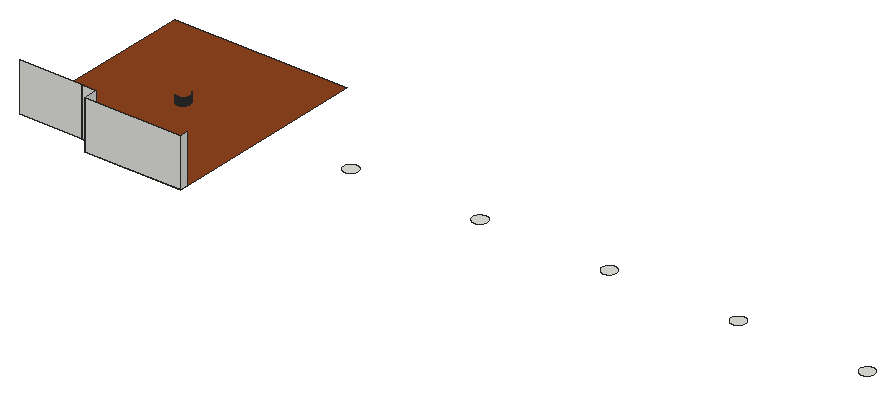
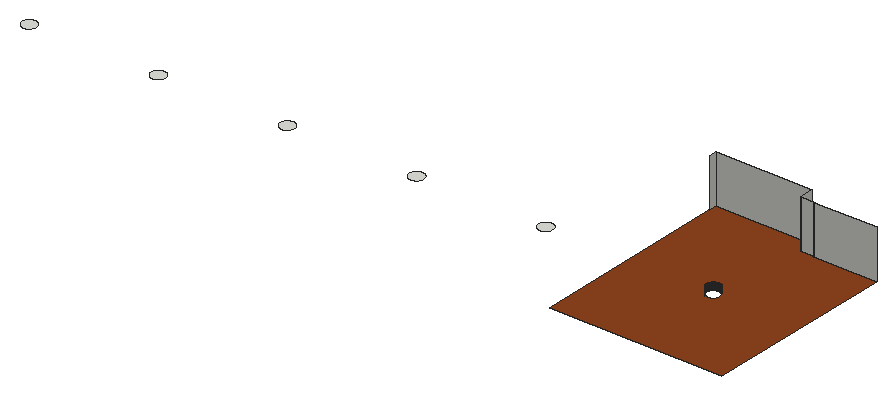
# SketchUp Ruby script. Lengths in inches.
U = 1.inch
M = Sketchup.active_model
def pt(a) = Geom::Point3d.new(a.map { |v| v * U })
def face(e, loops, mat)
  f = e.add_face(loops[0].map { |a| pt(a) })
  loops[1..].each { |l| e.add_face(l.map { |a| pt(a) }).erase! }
  f.material = f.back_material = mat if mat
  f
end
# faces: each face lists its corners as indices into pts; further lists are holes
def faces(e, pts, list, mat = nil) = list.each { |f| face(e, (f[0].is_a?(Array) ? f : [f]).map { |l| l.map { |i| pts[i] } }, mat) }
# xy, xz, yz: faces in a plane at the given z, y or x. An outline is a flat list of corners, or four numbers for a rectangle; further outlines are holes
def ring(l) = l.size == 4 ? [[l[0], l[1]], [l[2], l[1]], [l[2], l[3]], [l[0], l[3]]] : l.each_slice(2).to_a
def flat(e, list, mat, &to3) = list.each { |f| face(e, (f[0].is_a?(Array) ? f : [f]).map { |l| ring(l).map { |u, v| to3.(u, v) } }, mat) }
def xy(e, z, list, mat = nil) = flat(e, list, mat) { |x, y| [x, y, z] }
def xz(e, y, list, mat = nil) = flat(e, list, mat) { |x, z| [x, y, z] }
def yz(e, x, list, mat = nil) = flat(e, list, mat) { |y, z| [x, y, z] }
def lines(e, pts, list) = list.each { |a, b| e.add_line(pt(pts[a]), pt(pts[b])) }
# prism: a flat outline (further loops are holes) pulled along v
def prism(e, loops, v, mat = nil)
  f = face(e, loops, mat); d = Geom::Vector3d.new(v.map { |x| x * U })
  f.pushpull(f.normal.samedirection?(d) ? d.length : -d.length)
end
def box(e, o, s, mat = nil) = prism(e, [[o, [o[0] + s[0], o[1], o[2]], [o[0] + s[0], o[1] + s[1], o[2]], [o[0], o[1] + s[1], o[2]]]], [0, 0, s[2]], mat)
def at(x, y, z, deg = 0) = Geom::Transformation.translation(pt([x, y, z])) * Geom::Transformation.rotation(ORIGIN, Z_AXIS, deg.degrees)
def axes(o, x, y, z) = Geom::Transformation.new([*x, 0, *y, 0, *z, 0, *pt(o).to_a, 1])
def part(name) = M.definitions.add(name)
# library, detail: a bought-in or finely detailed component or shape, given as its bounding box
def library(name, o, s) = part(name).tap { |d| box(d.entities, o, s) }
def detail(e, o, s) = box(e.add_group.entities, o, s)
def put(e, d, t, mat = nil) = e.add_instance(d, t).tap { |i| i.material = mat if mat }
def group(e, t, mat = nil) = e.add_group.tap { |g| g.transformation = t; g.material = mat if mat }.entities
root = M.entities
M.materials.add("[Wood Fence]").color = [142, 67, 30]
xy(root,231,[[128.84,254,128.76,254.01,128.6875,254.02,128.61,254.03,128.45,254.05,128.375,254.07,128.3,254.08,128.22,254.1,128.15,254.125,128.07,254.15,128,254.17,127.92,254.2,127.71,254.29,127.64,254.33,127.57,254.36,127.43,254.44,127.37,254.48,127.3,254.53,127.24,254.57,127.17,254.62,126.93,254.82,126.88,254.88,126.82,254.93,126.62,255.17,126.57,255.24,126.53,255.3,126.48,255.37,126.44,255.43,126.36,255.57,126.33,255.64,126.29,255.71,126.2,255.92,126.17,256,126.15,256.07,126.125,256.15,126.1,256.22,126.08,256.3,126.07,256.375,126.05,256.45,126.03,256.61,126.02,256.6875,126.01,256.76,126,256.84,126,257.16,126.01,257.24,126.02,257.3125,126.03,257.39,126.05,257.55,126.07,257.625,126.08,257.7,126.1,257.78,126.125,257.85,126.15,257.93,126.17,258,126.2,258.08,126.29,258.29,126.33,258.36,126.36,258.43,126.44,258.57,126.48,258.63,126.53,258.7,126.57,258.76,126.62,258.83,126.82,259.07,126.88,259.12,126.93,259.18,127.17,259.38,127.24,259.43,127.3,259.47,127.37,259.52,127.43,259.56,127.57,259.64,127.64,259.67,127.71,259.71,127.92,259.8,128,259.83,128.07,259.85,128.15,259.875,128.22,259.9,128.3,259.92,128.375,259.93,128.45,259.95,128.61,259.97,128.6875,259.98,128.76,259.99,128.84,260,129.16,260,129.24,259.99,129.3125,259.98,129.39,259.97,129.55,259.95,129.625,259.93,129.7,259.92,129.78,259.9,129.85,259.875,129.93,259.85,130,259.83,130.08,259.8,130.29,259.71,130.36,259.67,130.43,259.64,130.57,259.56,130.63,259.52,130.7,259.47,130.76,259.43,130.83,259.38,131.07,259.18,131.12,259.12,131.18,259.07,131.38,258.83,131.43,258.76,131.47,258.7,131.52,258.63,131.56,258.57,131.64,258.43,131.67,258.36,131.71,258.29,131.8,258.08,131.83,258,131.85,257.93,131.875,257.85,131.9,257.78,131.92,257.7,131.93,257.625,131.95,257.55,131.97,257.39,131.98,257.3125,131.99,257.24,132,257.16,132,256.84,131.99,256.76,131.98,256.6875,131.97,256.61,131.95,256.45,131.93,256.375,131.92,256.3,131.9,256.22,131.875,256.15,131.85,256.07,131.83,256,131.8,255.92,131.71,255.71,131.67,255.64,131.64,255.57,131.56,255.43,131.52,255.37,131.47,255.3,131.43,255.24,131.38,255.17,131.18,254.93,131.12,254.88,131.07,254.82,130.83,254.62,130.76,254.57,130.7,254.53,130.63,254.48,130.57,254.44,130.43,254.36,130.36,254.33,130.29,254.29,130.08,254.2,130,254.17,129.93,254.15,129.85,254.125,129.78,254.1,129.7,254.08,129.625,254.07,129.55,254.05,129.39,254.03,129.3125,254.02,129.24,254.01,129.16,254],[184.84,254,184.76,254.01,184.6875,254.02,184.61,254.03,184.45,254.05,184.375,254.07,184.3,254.08,184.22,254.1,184.15,254.125,184.07,254.15,184,254.17,183.92,254.2,183.71,254.29,183.64,254.33,183.57,254.36,183.43,254.44,183.37,254.48,183.3,254.53,183.24,254.57,183.17,254.62,182.93,254.82,182.88,254.88,182.82,254.93,182.62,255.17,182.57,255.24,182.53,255.3,182.48,255.37,182.44,255.43,182.36,255.57,182.33,255.64,182.29,255.71,182.2,255.92,182.17,256,182.15,256.07,182.125,256.15,182.1,256.22,182.08,256.3,182.07,256.375,182.05,256.45,182.03,256.61,182.02,256.6875,182.01,256.76,182,256.84,182,257.16,182.01,257.24,182.02,257.3125,182.03,257.39,182.05,257.55,182.07,257.625,182.08,257.7,182.1,257.78,182.125,257.85,182.15,257.93,182.17,258,182.2,258.08,182.29,258.29,182.33,258.36,182.36,258.43,182.44,258.57,182.48,258.63,182.53,258.7,182.57,258.76,182.62,258.83,182.82,259.07,182.88,259.12,182.93,259.18,183.17,259.38,183.24,259.43,183.3,259.47,183.37,259.52,183.43,259.56,183.57,259.64,183.64,259.67,183.71,259.71,183.92,259.8,184,259.83,184.07,259.85,184.15,259.875,184.22,259.9,184.3,259.92,184.375,259.93,184.45,259.95,184.61,259.97,184.6875,259.98,184.76,259.99,184.84,260,185.16,260,185.24,259.99,185.3125,259.98,185.39,259.97,185.55,259.95,185.625,259.93,185.7,259.92,185.78,259.9,185.85,259.875,185.93,259.85,186,259.83,186.08,259.8,186.29,259.71,186.36,259.67,186.43,259.64,186.57,259.56,186.63,259.52,186.7,259.47,186.76,259.43,186.83,259.38,187.07,259.18,187.12,259.12,187.18,259.07,187.38,258.83,187.43,258.76,187.47,258.7,187.52,258.63,187.56,258.57,187.64,258.43,187.67,258.36,187.71,258.29,187.8,258.08,187.83,258,187.85,257.93,187.875,257.85,187.9,257.78,187.92,257.7,187.93,257.625,187.95,257.55,187.97,257.39,187.98,257.3125,187.99,257.24,188,257.16,188,256.84,187.99,256.76,187.98,256.6875,187.97,256.61,187.95,256.45,187.93,256.375,187.92,256.3,187.9,256.22,187.875,256.15,187.85,256.07,187.83,256,187.8,255.92,187.71,255.71,187.67,255.64,187.64,255.57,187.56,255.43,187.52,255.37,187.47,255.3,187.43,255.24,187.38,255.17,187.18,254.93,187.12,254.88,187.07,254.82,186.83,254.62,186.76,254.57,186.7,254.53,186.63,254.48,186.57,254.44,186.43,254.36,186.36,254.33,186.29,254.29,186.08,254.2,186,254.17,185.93,254.15,185.85,254.125,185.78,254.1,185.7,254.08,185.625,254.07,185.55,254.05,185.39,254.03,185.3125,254.02,185.24,254.01,185.16,254],[240.84,254,240.76,254.01,240.6875,254.02,240.61,254.03,240.45,254.05,240.375,254.07,240.3,254.08,240.22,254.1,240.15,254.125,240.07,254.15,240,254.17,239.92,254.2,239.71,254.29,239.64,254.33,239.57,254.36,239.43,254.44,239.37,254.48,239.3,254.53,239.24,254.57,239.17,254.62,238.93,254.82,238.88,254.88,238.82,254.93,238.62,255.17,238.57,255.24,238.53,255.3,238.48,255.37,238.44,255.43,238.36,255.57,238.33,255.64,238.29,255.71,238.2,255.92,238.17,256,238.15,256.07,238.125,256.15,238.1,256.22,238.08,256.3,238.07,256.375,238.05,256.45,238.03,256.61,238.02,256.6875,238.01,256.76,238,256.84,238,257.16,238.01,257.24,238.02,257.3125,238.03,257.39,238.05,257.55,238.07,257.625,238.08,257.7,238.1,257.78,238.125,257.85,238.15,257.93,238.17,258,238.2,258.08,238.29,258.29,238.33,258.36,238.36,258.43,238.44,258.57,238.48,258.63,238.53,258.7,238.57,258.76,238.62,258.83,238.82,259.07,238.88,259.12,238.93,259.18,239.17,259.38,239.24,259.43,239.3,259.47,239.37,259.52,239.43,259.56,239.57,259.64,239.64,259.67,239.71,259.71,239.92,259.8,240,259.83,240.07,259.85,240.15,259.875,240.22,259.9,240.3,259.92,240.375,259.93,240.45,259.95,240.61,259.97,240.6875,259.98,240.76,259.99,240.84,260,241.16,260,241.24,259.99,241.3125,259.98,241.39,259.97,241.55,259.95,241.625,259.93,241.7,259.92,241.78,259.9,241.85,259.875,241.93,259.85,242,259.83,242.08,259.8,242.29,259.71,242.36,259.67,242.43,259.64,242.57,259.56,242.63,259.52,242.7,259.47,242.76,259.43,242.83,259.38,243.07,259.18,243.12,259.12,243.18,259.07,243.38,258.83,243.43,258.76,243.47,258.7,243.52,258.63,243.56,258.57,243.64,258.43,243.67,258.36,243.71,258.29,243.8,258.08,243.83,258,243.85,257.93,243.875,257.85,243.9,257.78,243.92,257.7,243.93,257.625,243.95,257.55,243.97,257.39,243.98,257.3125,243.99,257.24,244,257.16,244,256.84,243.99,256.76,243.98,256.6875,243.97,256.61,243.95,256.45,243.93,256.375,243.92,256.3,243.9,256.22,243.875,256.15,243.85,256.07,243.83,256,243.8,255.92,243.71,255.71,243.67,255.64,243.64,255.57,243.56,255.43,243.52,255.37,243.47,255.3,243.43,255.24,243.38,255.17,243.18,254.93,243.12,254.88,243.07,254.82,242.83,254.62,242.76,254.57,242.7,254.53,242.63,254.48,242.57,254.44,242.43,254.36,242.36,254.33,242.29,254.29,242.08,254.2,242,254.17,241.93,254.15,241.85,254.125,241.78,254.1,241.7,254.08,241.625,254.07,241.55,254.05,241.39,254.03,241.3125,254.02,241.24,254.01,241.16,254],[296.84,254,296.76,254.01,296.6875,254.02,296.61,254.03,296.45,254.05,296.375,254.07,296.3,254.08,296.22,254.1,296.15,254.125,296.07,254.15,296,254.17,295.92,254.2,295.71,254.29,295.64,254.33,295.57,254.36,295.43,254.44,295.37,254.48,295.3,254.53,295.24,254.57,295.17,254.62,294.93,254.82,294.88,254.88,294.82,254.93,294.62,255.17,294.57,255.24,294.53,255.3,294.48,255.37,294.44,255.43,294.36,255.57,294.33,255.64,294.29,255.71,294.2,255.92,294.17,256,294.15,256.07,294.125,256.15,294.1,256.22,294.08,256.3,294.07,256.375,294.05,256.45,294.03,256.61,294.02,256.6875,294.01,256.76,294,256.84,294,257.16,294.01,257.24,294.02,257.3125,294.03,257.39,294.05,257.55,294.07,257.625,294.08,257.7,294.1,257.78,294.125,257.85,294.15,257.93,294.17,258,294.2,258.08,294.29,258.29,294.33,258.36,294.36,258.43,294.44,258.57,294.48,258.63,294.53,258.7,294.57,258.76,294.62,258.83,294.82,259.07,294.88,259.12,294.93,259.18,295.17,259.38,295.24,259.43,295.3,259.47,295.37,259.52,295.43,259.56,295.57,259.64,295.64,259.67,295.71,259.71,295.92,259.8,296,259.83,296.07,259.85,296.15,259.875,296.22,259.9,296.3,259.92,296.375,259.93,296.45,259.95,296.61,259.97,296.6875,259.98,296.76,259.99,296.84,260,297.16,260,297.24,259.99,297.3125,259.98,297.39,259.97,297.55,259.95,297.625,259.93,297.7,259.92,297.78,259.9,297.85,259.875,297.93,259.85,298,259.83,298.08,259.8,298.29,259.71,298.36,259.67,298.43,259.64,298.57,259.56,298.63,259.52,298.7,259.47,298.76,259.43,298.83,259.38,299.07,259.18,299.12,259.12,299.18,259.07,299.38,258.83,299.43,258.76,299.47,258.7,299.52,258.63,299.56,258.57,299.64,258.43,299.67,258.36,299.71,258.29,299.8,258.08,299.83,258,299.85,257.93,299.875,257.85,299.9,257.78,299.92,257.7,299.93,257.625,299.95,257.55,299.97,257.39,299.98,257.3125,299.99,257.24,300,257.16,300,256.84,299.99,256.76,299.98,256.6875,299.97,256.61,299.95,256.45,299.93,256.375,299.92,256.3,299.9,256.22,299.875,256.15,299.85,256.07,299.83,256,299.8,255.92,299.71,255.71,299.67,255.64,299.64,255.57,299.56,255.43,299.52,255.37,299.47,255.3,299.43,255.24,299.38,255.17,299.18,254.93,299.12,254.88,299.07,254.82,298.83,254.62,298.76,254.57,298.7,254.53,298.63,254.48,298.57,254.44,298.43,254.36,298.36,254.33,298.29,254.29,298.08,254.2,298,254.17,297.93,254.15,297.85,254.125,297.78,254.1,297.7,254.08,297.625,254.07,297.55,254.05,297.39,254.03,297.3125,254.02,297.24,254.01,297.16,254],[352.84,254,352.76,254.01,352.6875,254.02,352.61,254.03,352.45,254.05,352.375,254.07,352.3,254.08,352.22,254.1,352.15,254.125,352.07,254.15,352,254.17,351.92,254.2,351.71,254.29,351.64,254.33,351.57,254.36,351.43,254.44,351.37,254.48,351.3,254.53,351.24,254.57,351.17,254.62,350.93,254.82,350.88,254.88,350.82,254.93,350.62,255.17,350.57,255.24,350.53,255.3,350.48,255.37,350.44,255.43,350.36,255.57,350.33,255.64,350.29,255.71,350.2,255.92,350.17,256,350.15,256.07,350.125,256.15,350.1,256.22,350.08,256.3,350.07,256.375,350.05,256.45,350.03,256.61,350.02,256.6875,350.01,256.76,350,256.84,350,257.16,350.01,257.24,350.02,257.3125,350.03,257.39,350.05,257.55,350.07,257.625,350.08,257.7,350.1,257.78,350.125,257.85,350.15,257.93,350.17,258,350.2,258.08,350.29,258.29,350.33,258.36,350.36,258.43,350.44,258.57,350.48,258.63,350.53,258.7,350.57,258.76,350.62,258.83,350.82,259.07,350.88,259.12,350.93,259.18,351.17,259.38,351.24,259.43,351.3,259.47,351.37,259.52,351.43,259.56,351.57,259.64,351.64,259.67,351.71,259.71,351.92,259.8,352,259.83,352.07,259.85,352.15,259.875,352.22,259.9,352.3,259.92,352.375,259.93,352.45,259.95,352.61,259.97,352.6875,259.98,352.76,259.99,352.84,260,353.16,260,353.24,259.99,353.3125,259.98,353.39,259.97,353.55,259.95,353.625,259.93,353.7,259.92,353.78,259.9,353.85,259.875,353.93,259.85,354,259.83,354.08,259.8,354.29,259.71,354.36,259.67,354.43,259.64,354.57,259.56,354.63,259.52,354.7,259.47,354.76,259.43,354.83,259.38,355.07,259.18,355.12,259.12,355.18,259.07,355.38,258.83,355.43,258.76,355.47,258.7,355.52,258.63,355.56,258.57,355.64,258.43,355.67,258.36,355.71,258.29,355.8,258.08,355.83,258,355.85,257.93,355.875,257.85,355.9,257.78,355.92,257.7,355.93,257.625,355.95,257.55,355.97,257.39,355.98,257.3125,355.99,257.24,356,257.16,356,256.84,355.99,256.76,355.98,256.6875,355.97,256.61,355.95,256.45,355.93,256.375,355.92,256.3,355.9,256.22,355.875,256.15,355.85,256.07,355.83,256,355.8,255.92,355.71,255.71,355.67,255.64,355.64,255.57,355.56,255.43,355.52,255.37,355.47,255.3,355.43,255.24,355.38,255.17,355.18,254.93,355.12,254.88,355.07,254.82,354.83,254.62,354.76,254.57,354.7,254.53,354.63,254.48,354.57,254.44,354.43,254.36,354.36,254.33,354.29,254.29,354.08,254.2,354,254.17,353.93,254.15,353.85,254.125,353.78,254.1,353.7,254.08,353.625,254.07,353.55,254.05,353.39,254.03,353.3125,254.02,353.24,254.01,353.16,254]])
xy(root,231,[[[51,210,51,216,45,216,45,216.5,18,216.5,18,300,93,300,93,210],[55.37,255,55.6,255,55.68,255.01,55.76,255.01,55.92,255.03,55.99,255.04,56.07,255.05,56.15,255.07,56.22,255.09,56.3,255.11,56.45,255.15,56.53,255.18,56.74,255.27,56.8125,255.3,56.88,255.34,57.02,255.41,57.09,255.46,57.16,255.5,57.22,255.54,57.28,255.59,57.35,255.64,57.41,255.68,57.47,255.74,57.53,255.79,57.75,256.01,57.9,256.19,57.94,256.26,57.99,256.32,58.03,256.39,58.07,256.45,58.15,256.59,58.18,256.66,58.22,256.73,58.25,256.8,58.31,256.95,58.34,257.02,58.36,257.1,58.38,257.17,58.4,257.25,58.42,257.32,58.44,257.4,58.45,257.48,58.47,257.56,58.48,257.63,58.49,257.71,58.49,257.79,58.5,257.87,58.5,258.1,58.49,258.18,58.49,258.26,58.47,258.42,58.46,258.49,58.45,258.57,58.43,258.65,58.41,258.72,58.39,258.8,58.35,258.95,58.32,259.03,58.23,259.24,58.2,259.3125,58.16,259.38,58.09,259.52,58.04,259.59,58,259.66,57.96,259.72,57.91,259.78,57.86,259.85,57.82,259.91,57.76,259.97,57.71,260.03,57.49,260.25,57.31,260.4,57.24,260.44,57.18,260.49,57.11,260.53,57.05,260.57,56.91,260.65,56.84,260.68,56.77,260.72,56.7,260.75,56.55,260.81,56.48,260.84,56.4,260.86,56.33,260.88,56.25,260.9,56.18,260.92,56.1,260.94,56.02,260.95,55.94,260.97,55.87,260.98,55.79,260.99,55.71,260.99,55.63,261,55.4,261,55.32,260.99,55.24,260.99,55.08,260.97,55.01,260.96,54.93,260.95,54.85,260.93,54.78,260.91,54.7,260.89,54.55,260.85,54.47,260.82,54.26,260.73,54.1875,260.7,54.12,260.66,53.98,260.59,53.91,260.54,53.84,260.5,53.78,260.46,53.72,260.41,53.65,260.36,53.59,260.32,53.53,260.26,53.47,260.21,53.25,259.99,53.1,259.81,53.06,259.74,53.01,259.68,52.97,259.61,52.93,259.55,52.85,259.41,52.82,259.34,52.78,259.27,52.75,259.2,52.69,259.05,52.66,258.98,52.64,258.9,52.62,258.83,52.6,258.75,52.58,258.68,52.56,258.6,52.55,258.52,52.53,258.44,52.52,258.37,52.51,258.29,52.51,258.21,52.5,258.13,52.5,257.9,52.51,257.82,52.51,257.74,52.53,257.58,52.54,257.51,52.55,257.43,52.57,257.35,52.59,257.28,52.61,257.2,52.65,257.05,52.68,256.97,52.77,256.76,52.8,256.6875,52.84,256.62,52.91,256.48,52.96,256.41,53,256.34,53.04,256.28,53.09,256.22,53.14,256.15,53.18,256.09,53.24,256.03,53.29,255.97,53.51,255.75,53.69,255.6,53.76,255.56,53.82,255.51,53.89,255.47,53.95,255.43,54.09,255.35,54.16,255.32,54.23,255.28,54.3,255.25,54.45,255.19,54.52,255.16,54.6,255.14,54.67,255.12,54.75,255.1,54.82,255.08,54.9,255.06,54.98,255.05,55.06,255.03,55.13,255.02,55.21,255.01,55.29,255.01]]],"[Wood Fence]")
xz(root,210,[[51,231,93,252]])
xz(root,216,[[45,231,51,252]])
xz(root,216.5,[[18,231,45,252]])
xz(root,255,[[55.37,231,55.45,234],[55.45,231,55.53,234],[55.53,231,55.6,234]],"[Wood Fence]")
xz(root,255.01,[[55.21,231,55.29,234],[55.68,231,55.76,234]],"[Wood Fence]")
yz(root,45,[[216,231,216.5,252]])
yz(root,51,[[210,231,216,252]])
yz(root,58.49,[[257.71,231,257.79,234],[258.18,231,258.26,234]],"[Wood Fence]")
yz(root,58.5,[[257.87,231,257.95,234],[257.95,231,258.03,234],[258.03,231,258.1,234]],"[Wood Fence]")
yz(root,93,[[210,231,213,252]])
p = [[54.98,255.05,231],[54.9,255.06,231],[54.9,255.06,234],[54.98,255.05,234],[55.06,255.03,231],[55.06,255.03,234],
  [55.21,255.01,231],[55.13,255.02,231],[55.13,255.02,234],[55.21,255.01,234],[55.37,255,231],[55.29,255.01,231],
  [55.29,255.01,234],[55.37,255,234],[55.68,255.01,231],[55.6,255,231],[55.6,255,234],[55.68,255.01,234],
  [55.92,255.03,231],[55.84,255.02,231],[55.84,255.02,234],[55.92,255.03,234],[55.76,255.01,231],[55.76,255.01,234],
  [55.99,255.04,231],[55.99,255.04,234],[56.07,255.05,231],[56.07,255.05,234],[54.6,255.14,231],[54.52,255.16,231],
  [54.52,255.16,234],[54.6,255.14,234],[54.67,255.12,231],[54.67,255.12,234],[54.82,255.08,231],[54.75,255.1,231],
  [54.75,255.1,234],[54.82,255.08,234],[56.22,255.09,231],[56.15,255.07,231],[56.15,255.07,234],[56.22,255.09,234],
  [56.3,255.11,231],[56.3,255.11,234],[56.375,255.13,231],[56.375,255.13,234],[56.45,255.15,231],[56.45,255.15,234],
  [54.3,255.25,231],[54.23,255.28,231],[54.23,255.28,234],[54.3,255.25,234],[54.375,255.22,231],[54.375,255.22,234],
  [54.45,255.19,231],[54.45,255.19,234],[56.6,255.21,231],[56.53,255.18,231],[56.53,255.18,234],[56.6,255.21,234],
  [56.67,255.24,231],[56.67,255.24,234],[56.74,255.27,231],[56.74,255.27,234],[54.16,255.32,231],[54.09,255.35,231],
  [54.09,255.35,234],[54.16,255.32,234],[56.8125,255.3,231],[56.8125,255.3,234],[56.88,255.34,231],[56.88,255.34,234],
  [56.95,255.375,231],[56.95,255.375,234],[53.95,255.43,231],[53.89,255.47,231],[53.89,255.47,234],[53.95,255.43,234],
  [54.02,255.39,231],[54.02,255.39,234],[57.09,255.46,231],[57.02,255.41,231],[57.02,255.41,234],[57.09,255.46,234],
  [53.82,255.51,231],[53.82,255.51,234],[53.76,255.56,231],[53.76,255.56,234],[57.16,255.5,231],[57.16,255.5,234],
  [57.28,255.59,231],[57.22,255.54,231],[57.22,255.54,234],[57.28,255.59,234],[53.69,255.6,231],[53.63,255.65,231],
  [53.63,255.65,234],[53.69,255.6,234],[57.41,255.68,231],[57.35,255.64,231],[57.35,255.64,234],[57.41,255.68,234],
  [53.57,255.7,231],[53.57,255.7,234],[57.47,255.74,231],[57.47,255.74,234],[57.53,255.79,231],[57.53,255.79,234],
  [57.58,255.84,231],[57.58,255.84,234],[57.64,255.9,231],[57.64,255.9,234],[57.69,255.95,231],[57.69,255.95,234],
  [57.8,256.07,231],[57.75,256.01,231],[57.75,256.01,234],[57.8,256.07,234],[57.9,256.19,231],[57.85,256.13,231],
  [57.85,256.13,234],[57.9,256.19,234],[57.94,256.26,231],[57.94,256.26,234],[57.99,256.32,231],[57.99,256.32,234],
  [58.03,256.39,231],[58.03,256.39,234],[58.07,256.45,231],[58.07,256.45,234],[58.15,256.59,231],[58.11,256.52,231],
  [58.11,256.52,234],[58.15,256.59,234],[58.18,256.66,231],[58.18,256.66,234],[58.25,256.8,231],[58.22,256.73,231],
  [58.22,256.73,234],[58.25,256.8,234],[58.28,256.875,231],[58.28,256.875,234],[58.34,257.02,231],[58.31,256.95,231],
  [58.31,256.95,234],[58.34,257.02,234],[58.36,257.1,231],[58.36,257.1,234],[58.38,257.17,231],[58.38,257.17,234],
  [58.42,257.32,231],[58.4,257.25,231],[58.4,257.25,234],[58.42,257.32,234],[58.44,257.4,231],[58.44,257.4,234],
  [58.45,257.48,231],[58.45,257.48,234],[58.47,257.56,231],[58.47,257.56,234],[58.49,257.71,231],[58.48,257.63,231],
  [58.48,257.63,234],[58.49,257.71,234],[58.5,257.87,231],[58.49,257.79,231],[58.49,257.79,234],[58.5,257.87,234],
  [58.49,258.18,231],[58.5,258.1,231],[58.5,258.1,234],[58.49,258.18,234],[58.47,258.42,231],[58.48,258.34,231],
  [58.48,258.34,234],[58.47,258.42,234],[58.49,258.26,231],[58.49,258.26,234],[58.46,258.49,231],[58.46,258.49,234],
  [58.45,258.57,231],[58.45,258.57,234],[58.41,258.72,231],[58.43,258.65,231],[58.43,258.65,234],[58.41,258.72,234],
  [58.39,258.8,231],[58.39,258.8,234],[58.37,258.875,231],[58.37,258.875,234],[58.35,258.95,231],[58.35,258.95,234],
  [58.29,259.1,231],[58.32,259.03,231],[58.32,259.03,234],[58.29,259.1,234],[58.26,259.17,231],[58.26,259.17,234],
  [58.2,259.3125,231],[58.23,259.24,231],[58.23,259.24,234],[58.2,259.3125,234],[58.16,259.38,231],[58.16,259.38,234],
  [58.125,259.45,231],[58.125,259.45,234],[58.04,259.59,231],[58.09,259.52,231],[58.09,259.52,234],[58.04,259.59,234],
  [58,259.66,231],[58,259.66,234],[57.91,259.78,231],[57.96,259.72,231],[57.96,259.72,234],[57.91,259.78,234],
  [57.82,259.91,231],[57.86,259.85,231],[57.86,259.85,234],[57.82,259.91,234],[57.76,259.97,231],[57.76,259.97,234],
  [57.66,260.08,231],[57.71,260.03,231],[57.71,260.03,234],[57.66,260.08,234],[57.55,260.19,231],[57.6,260.14,231],
  [57.6,260.14,234],[57.55,260.19,234],[57.43,260.3,231],[57.49,260.25,231],[57.49,260.25,234],[57.43,260.3,234],
  [57.31,260.4,231],[57.37,260.35,231],[57.37,260.35,234],[57.31,260.4,234],[57.18,260.49,231],[57.24,260.44,231],
  [57.24,260.44,234],[57.18,260.49,234],[57.11,260.53,231],[57.11,260.53,234]]
faces(root,p,[[0,1,2,3],[4,0,3,5],[6,7,8,9],[7,4,5,8],[10,11,12,13],[14,15,16,17],[18,19,20,21],[19,22,23,20],
  [24,18,21,25],[26,24,25,27],[28,29,30,31],[32,28,31,33],[34,35,36,37],[35,32,33,36],[1,34,37,2],[38,39,40,41],
  [39,26,27,40],[42,38,41,43],[44,42,43,45],[46,44,45,47],[48,49,50,51],[52,48,51,53],[29,54,55,30],[54,52,53,55],
  [56,57,58,59],[57,46,47,58],[60,56,59,61],[62,60,61,63],[64,65,66,67],[49,64,67,50],[68,62,63,69],[70,68,69,71],
  [72,70,71,73],[74,75,76,77],[65,78,79,66],[78,74,77,79],[80,81,82,83],[81,72,73,82],[75,84,85,76],[84,86,87,85],
  [88,80,83,89],[90,91,92,93],[91,88,89,92],[94,95,96,97],[86,94,97,87],[98,99,100,101],[99,90,93,100],[95,102,103,96],
  [104,98,101,105],[106,104,105,107],[108,106,107,109],[110,108,109,111],[112,110,111,113],[114,115,116,117],[115,112,113,116],[118,119,120,121],
  [119,114,117,120],[122,118,121,123],[124,122,123,125],[126,124,125,127],[128,126,127,129],[130,131,132,133],[131,128,129,132],[134,130,133,135],
  [136,137,138,139],[137,134,135,138],[140,136,139,141],[142,143,144,145],[143,140,141,144],[146,142,145,147],[148,146,147,149],[150,151,152,153],
  [151,148,149,152],[154,150,153,155],[156,154,155,157],[158,156,157,159],[160,161,162,163],[161,158,159,162],[164,165,166,167],[168,169,170,171],
  [172,173,174,175],[173,176,177,174],[178,172,175,179],[180,178,179,181],[182,183,184,185],[183,180,181,184],[186,182,185,187],[188,186,187,189],
  [190,188,189,191],[192,193,194,195],[193,190,191,194],[196,192,195,197],[198,199,200,201],[199,196,197,200],[202,198,201,203],[204,202,203,205],
  [206,207,208,209],[207,204,205,208],[210,206,209,211],[212,213,214,215],[213,210,211,214],[216,217,218,219],[217,212,215,218],[220,216,219,221],
  [222,223,224,225],[223,220,221,224],[226,227,228,229],[227,222,225,228],[230,231,232,233],[231,226,229,232],[234,235,236,237],[235,230,233,236],
  [238,239,240,241],[239,234,237,240],[242,238,241,243]],"[Wood Fence]")
